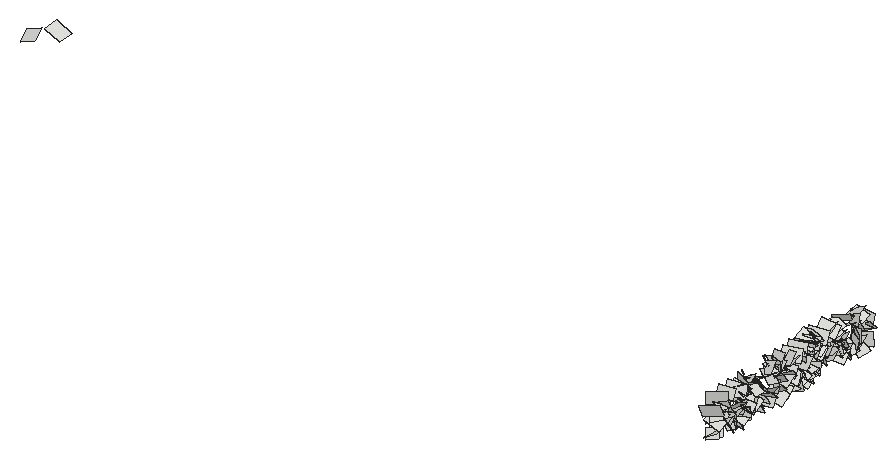
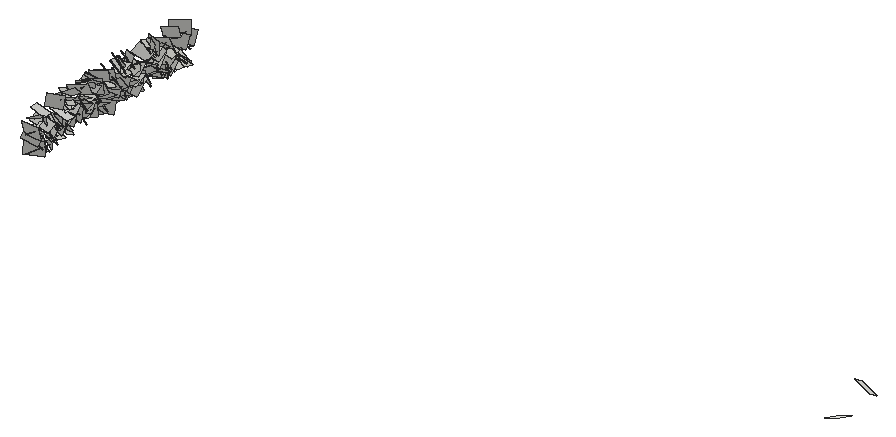
# SketchUp Ruby script. Lengths in inches.
U = 1.inch
M = Sketchup.active_model
def pt(a) = Geom::Point3d.new(a.map { |v| v * U })
def face(e, loops, mat)
  f = e.add_face(loops[0].map { |a| pt(a) })
  loops[1..].each { |l| e.add_face(l.map { |a| pt(a) }).erase! }
  f.material = f.back_material = mat if mat
  f
end
# faces: each face lists its corners as indices into pts; further lists are holes
def faces(e, pts, list, mat = nil) = list.each { |f| face(e, (f[0].is_a?(Array) ? f : [f]).map { |l| l.map { |i| pts[i] } }, mat) }
# xy, xz, yz: faces in a plane at the given z, y or x. An outline is a flat list of corners, or four numbers for a rectangle; further outlines are holes
def ring(l) = l.size == 4 ? [[l[0], l[1]], [l[2], l[1]], [l[2], l[3]], [l[0], l[3]]] : l.each_slice(2).to_a
def flat(e, list, mat, &to3) = list.each { |f| face(e, (f[0].is_a?(Array) ? f : [f]).map { |l| ring(l).map { |u, v| to3.(u, v) } }, mat) }
def xy(e, z, list, mat = nil) = flat(e, list, mat) { |x, y| [x, y, z] }
def xz(e, y, list, mat = nil) = flat(e, list, mat) { |x, z| [x, y, z] }
def yz(e, x, list, mat = nil) = flat(e, list, mat) { |y, z| [x, y, z] }
def lines(e, pts, list) = list.each { |a, b| e.add_line(pt(pts[a]), pt(pts[b])) }
# prism: a flat outline (further loops are holes) pulled along v
def prism(e, loops, v, mat = nil)
  f = face(e, loops, mat); d = Geom::Vector3d.new(v.map { |x| x * U })
  f.pushpull(f.normal.samedirection?(d) ? d.length : -d.length)
end
def box(e, o, s, mat = nil) = prism(e, [[o, [o[0] + s[0], o[1], o[2]], [o[0] + s[0], o[1] + s[1], o[2]], [o[0], o[1] + s[1], o[2]]]], [0, 0, s[2]], mat)
def at(x, y, z, deg = 0) = Geom::Transformation.translation(pt([x, y, z])) * Geom::Transformation.rotation(ORIGIN, Z_AXIS, deg.degrees)
def axes(o, x, y, z) = Geom::Transformation.new([*x, 0, *y, 0, *z, 0, *pt(o).to_a, 1])
def part(name) = M.definitions.add(name)
# library, detail: a bought-in or finely detailed component or shape, given as its bounding box
def library(name, o, s) = part(name).tap { |d| box(d.entities, o, s) }
def detail(e, o, s) = box(e.add_group.entities, o, s)
def put(e, d, t, mat = nil) = e.add_instance(d, t).tap { |i| i.material = mat if mat }
def group(e, t, mat = nil) = e.add_group.tap { |g| g.transformation = t; g.material = mat if mat }.entities
root = M.entities
c1 = part("Component\#6")
p = [[0.01,0,0],[0,3.24,4.54],[4.32,3.24,4.54],[4.33,0,0]]
faces(c1.entities,p,[[0,1,2,3]])
put(root,c1,axes([34.14,183.19,37.72],[0.19709,-1.17807,-0.70591],[0.26547,-0.67132,1.18631],[1.43137,0.28672,-0.12282]))
put(root,c1,axes([34.14,193.54,33.12],[0.22081,1.30446,0.31828],[0.37279,0.25784,-1.28691],[1.3736,-0.27967,0.29809]))
put(root,c1,axes([404.88,193.54,33.12],[-0.22081,1.30446,0.31828],[-0.37279,0.25784,-1.28691],[-1.3736,-0.27967,0.29809]))
put(root,c1,axes([404.88,183.19,37.72],[-0.19709,-1.17807,-0.70591],[-0.26547,-0.67132,1.18631],[-1.43137,0.28672,-0.12282]))
put(root,c1,axes([404.88,179.625,37.91],[-0.28026,0.12179,-1.29213],[-0.26115,-1.29941,-0.07206],[-1.35072,0.22596,0.28204]))
put(root,c1,axes([404.88,128.43,31.91],[-0.33386,1.00192,0.91989],[-0.02581,0.93993,-1.03208],[-1.44154,-0.24887,-0.19457]))
put(root,c1,axes([404.88,132.63,34.3],[-0.186,1.33026,-0.17859],[-0.24164,-0.20703,-1.31812],[-1.40205,-0.1408,0.25087]))
put(root,c1,axes([404.88,206.12,25.83],[-0.28838,0.48251,1.20317],[-0.13396,1.21365,-0.51529],[-1.36755,-0.22063,-0.20324]))
put(root,c1,axes([404.88,163.2,33.68],[-0.16473,-1.2102,0.57798],[-0.2383,0.59712,1.18983],[-1.40149,0.04071,-0.27024]))
put(root,c1,axes([404.88,132.49,21.15],[-0.19066,-0.73145,1.17679],[-0.11238,1.19045,0.72374],[-1.46442,0.00387,-0.20876]))
put(root,c1,axes([404.88,205.05,35.75],[-0.23328,1.34713,-0.22992],[-0.05022,-0.24027,-1.36238],[-1.44774,-0.20874,0.08431]))
put(root,c1,axes([405.22,214.11,35.21],[-0.07772,-0.27644,-1.33377],[-0.91911,-1.02064,0.2592],[-1.11351,0.86175,-0.12086]))
put(root,c1,axes([404.88,141,38.04],[-0.14868,1.2474,-0.57055],[-0.09146,-0.58042,-1.24775],[-1.45112,-0.09122,0.1371]))
put(root,c1,axes([405.59,124.93,30.08],[-0.69154,0.83647,0.57299],[-0.50453,0.34895,-1.05134],[-0.94895,-0.79509,0.14141]))
put(root,c1,axes([404.88,153.14,23.91],[-0.18,-1.08552,0.79109],[-0.08355,0.80406,1.08641],[-1.42134,0.0902,-0.16405]))
put(root,c1,axes([404.88,190.14,35.27],[-0.30668,1.10496,-0.445],[-0.14325,-0.48543,-1.11748],[-1.25452,-0.21469,0.23639]))
put(root,c1,axes([404.88,186.51,25.44],[0.00901,-0.3677,1.34811],[-0.26845,1.32541,0.3631],[-1.45667,-0.24653,-0.05858]))
put(root,c1,axes([404.88,195.625,24.52],[-0.22176,-0.47224,1.18941],[-0.10161,1.2076,0.46259],[-1.3527,-0.0133,-0.22974]))
put(root,c1,axes([404.88,143.09,24.72],[-0.05768,-1.1082,-0.74759],[-0.23067,-0.73089,1.09928],[-1.3981,0.16631,-0.15052]))
put(root,c1,axes([404.88,205.51,24.88],[-0.13882,1.11155,0.63897],[-0.19603,0.6192,-1.11507],[-1.34484,-0.205,0.09658]))
put(root,c1,axes([404.88,157.9,37.93],[-0.24747,1.3445,0.30187],[0.11522,0.32319,-1.35538],[-1.4561,-0.20293,-0.15855]))
put(root,c1,axes([404.88,137.42,26.21],[-0.14568,0.69276,1.17725],[-0.03045,1.18146,-0.69859],[-1.44759,-0.09457,-0.10377]))
put(root,c1,axes([404.88,213.57,27.56],[0.01798,0.03957,-1.39555],[-0.22262,-1.3797,-0.04168],[-1.46303,0.21042,-0.01081]))
put(root,c1,axes([404.88,168.45,29.92],[-0.2904,-0.81126,-1.09363],[0.15157,-1.12651,0.79984],[-1.4354,0.04517,0.30571]))
put(root,c1,axes([404.88,159.18,36.25],[-0.04304,0.74935,1.15311],[-0.14712,1.14549,-0.74928],[-1.45028,-0.13844,0.04179]))
put(root,c1,axes([404.88,165.11,34.6875],[-0.03998,0.77126,1.05992],[-0.2457,1.03973,-0.76482],[-1.36759,-0.20934,0.10642]))
put(root,c1,axes([404.88,200.57,23.13],[-0.2198,-0.69796,1.13548],[0.0671,1.14269,0.71395],[-1.41122,0.16304,-0.1429]))
put(root,c1,axes([404.88,153.125,28.17],[0.03085,-0.9293,0.97672],[-0.26234,0.95667,0.91759],[-1.40479,-0.19906,-0.14991]))
put(root,c1,axes([404.88,172.42,21.79],[-0.22827,-1.35966,0.24048],[0.1567,0.21929,1.3722],[-1.45519,0.2369,0.11004]))
put(root,c1,axes([404.88,122.33,25.2],[-0.14417,1.26196,0.33106],[-0.05821,0.32703,-1.26913],[-1.38172,-0.14545,0.01892]))
put(root,c1,axes([404.88,127.05,26.22],[-0.14417,1.26196,0.33106],[-0.05821,0.32703,-1.26913],[-1.38172,-0.14545,0.01892]))
put(root,c1,axes([404.88,177.28,39.83],[-0.04784,1.11638,-0.64936],[-0.22797,-0.64718,-1.09769],[-1.34988,0.06974,0.20839]))
put(root,c1,axes([404.93,125.55,22.43],[-0.36857,0.54861,0.76203],[-0.54406,0.56941,-0.64413],[-0.83345,-0.61431,0.08349]))
put(root,c1,axes([404.93,123.49,22.43],[-0.36857,0.54861,0.76203],[-0.54406,0.56941,-0.64413],[-0.83345,-0.61431,0.08349]))
put(root,c1,axes([404.88,153.73,28.3],[0.01858,0.99462,-0.84655],[-0.29457,-0.8244,-0.97435],[-1.35277,0.19318,0.20054]))
put(root,c1,axes([404.88,128.45,36.29],[0.02149,0.52903,-1.24729],[-0.2007,-1.23408,-0.5265],[-1.42204,0.18216,0.05546]))
put(root,c1,axes([404.88,124,36.29],[0.02149,0.52903,-1.24729],[-0.2007,-1.23408,-0.5265],[-1.42204,0.18216,0.05546]))
put(root,c1,axes([404.88,128.47,40.0625],[-0.15368,0.21217,-1.35934],[0.08132,-1.3635,-0.221],[-1.45608,-0.09854,0.13113]))
put(root,c1,axes([404.88,188.1875,39.24],[-0.00053,-0.50504,-1.25708],[-0.1621,-1.24903,0.50186],[-1.42684,0.14209,-0.05655]))
put(root,c1,axes([404.88,199.97,41.09],[-0.2759,0.65189,-0.94787],[-0.07756,-0.97924,-0.65337],[-1.21695,-0.08538,0.25653]))
put(root,c1,axes([404.88,183.77,26.5],[-0.0762,-1.33255,-0.21023],[-0.04546,-0.20817,1.33413],[-1.42926,0.07766,-0.03122]))
put(root,c1,axes([404.88,140.4,37.84],[0.00777,-0.46206,-1.23937],[-0.21731,-1.22481,0.45542],[-1.38512,0.18957,-0.0784]))
put(root,c1,axes([404.88,193.84,30.46],[-0.25587,-1.06575,0.3461],[-0.15582,0.3811,1.07099],[-1.17751,0.18115,-0.21693]))
put(root,c1,axes([404.88,194.52,25.48],[-0.11423,-0.20624,1.26777],[-0.06819,1.2715,0.20138],[-1.3598,-0.04643,-0.1166]))
put(root,c1,axes([404.88,189.88,26.35],[-0.12674,1.17916,0.69894],[0.07675,0.70605,-1.17877],[-1.45096,-0.06565,-0.1234]))
put(root,c1,axes([404.88,142.63,35.02],[-0.11092,-0.98462,-0.77371],[-0.1183,-0.76598,0.98988],[-1.32209,0.15114,-0.02366]))
put(root,c1,axes([404.88,142.42,32.89],[-0.18672,-0.42722,1.28431],[0.1337,1.28432,0.44452],[-1.42847,0.17605,-0.12627]))
put(root,c1,axes([404.88,177.96,25.04],[-0.10915,-1.1796,-0.55067],[-0.03689,-0.5497,1.18402],[-1.37942,0.10803,0.01191]))
put(root,c1,axes([404.88,133.32,22.11],[-0.03082,0.0656,1.39488],[0.001,1.39518,-0.0656],[-1.48021,-0.00042,-0.02909]))
put(root,c1,axes([404.88,161.74,34.71],[-0.1652,-1.10091,-0.16395],[-0.26327,-0.12698,1.08875],[-1.15009,0.1872,-0.22568]))
put(root,c1,axes([404.88,211.92,20.51],[-0.20622,-1.25394,-0.15944],[0.06822,-0.17093,1.26581],[-1.33814,0.18453,0.0891]))
put(root,c1,axes([404.88,204.65,33.57],[-0.11682,0.36237,1.1463],[-0.15256,1.13885,-0.37385],[-1.26518,-0.17079,-0.06076]))
put(root,c1,axes([404.88,157.5625,26.25],[-0.15158,-0.38022,-1.22414],[0.0526,-1.23246,0.37701],[-1.35773,-0.0053,0.15127]))
put(root,c1,axes([404.88,135.17,32.61],[-0.12448,1.21649,-0.63228],[0.14654,-0.62086,-1.22019],[-1.44585,-0.16766,-0.06923]))
put(root,c1,axes([404.88,175.66,39.88],[0.03914,-0.32872,-1.22009],[-0.25418,-1.20026,0.31612],[-1.31508,0.2222,-0.09741]))
put(root,c1,axes([404.88,205.46,24.09],[-0.08024,0.04196,1.34674],[0.06239,1.34768,-0.03868],[-1.42687,0.05657,-0.07742]))
put(root,c1,axes([404.88,158.06,26.05],[-0.19995,0.52409,1.06255],[-0.00833,1.07535,-0.5318],[-1.25583,-0.09057,-0.16565]))
put(root,c1,axes([404.88,166.62,31.96],[-0.21061,0.75098,-0.921],[0.02022,-0.93165,-0.76377],[-1.25951,-0.14053,0.14175]))
put(root,c1,axes([404.88,139.39,34.34],[-0.15089,0.92592,0.71699],[-0.08883,0.71236,-0.93659],[-1.23815,-0.16395,-0.02018]))
put(root,c1,axes([404.88,196.54,35.06],[-0.17609,-1.11494,-0.45613],[0.00034,-0.46049,1.12547],[-1.27691,0.15363,0.0632]))
put(root,c1,axes([404.88,156.14,33.68],[-0.06217,-0.55405,1.15944],[-0.03014,1.16092,0.55332],[-1.36179,-0.0004,-0.06518]))
put(root,c1,axes([404.88,205.63,39.17],[-0.17317,1.06099,0.10432],[-0.22006,0.07185,-1.05594],[-1.10844,-0.18002,0.19334]))
put(root,c1,axes([404.88,153.92,36.42],[-0.14295,0.82362,0.79821],[-0.11339,0.79118,-0.83443],[-1.21047,-0.17138,-0.0161]))
put(root,c1,axes([404.88,140.25,33.3],[0.10371,-0.10781,1.29757],[-0.22808,1.282,0.12274],[-1.36119,-0.22303,0.07829]))
put(root,c1,axes([404.88,180.73,30.67],[-0.05707,0.69485,1.12415],[0.04583,1.1254,-0.69356],[-1.4001,0.00851,-0.06852]))
put(root,c1,axes([404.88,145.83,38.68],[0.04371,1.09164,-0.51046],[-0.28885,-0.48908,-1.06793],[-1.24431,0.15188,0.22998]))
put(root,c1,axes([404.88,199.72,26.12],[0.08735,-0.8928,-1.02237],[-0.07635,-1.02569,0.88989],[-1.43674,0.00023,-0.10945]))
put(root,c1,axes([404.88,169.91,24.28],[0.0494,0.58776,1.07494],[-0.25393,1.05932,-0.56884],[-1.27358,-0.18841,0.15511]))
put(root,c1,axes([404.88,178.68,21.25],[-0.14964,-1.02559,0.91665],[0.24358,0.89093,1.03221],[-1.43757,0.25771,0.07948]))
put(root,c1,axes([404.88,196.35,30.1],[-0.25467,1.00338,0.64071],[0.12934,0.67094,-1.00496],[-1.25528,-0.13443,-0.23354]))
put(root,c1,axes([404.88,158.99,33.95],[-0.09747,0.08794,1.12692],[-0.17247,1.11783,-0.1005],[-1.18568,-0.16983,-0.07802]))
put(root,c1,axes([404.88,188.72,38.18],[-0.108,1.17484,0.54266],[0.09899,0.5496,-1.17232],[-1.36819,-0.05298,-0.12766]))
put(root,c1,axes([404.88,187.26,33.24],[-0.066,-0.95024,-0.64083],[-0.19237,-0.6255,0.94515],[-1.19957,0.15259,-0.11631]))
put(root,c1,axes([404.88,141.15,27.9],[-0.10356,0.25866,-1.08582],[-0.18317,-1.08033,-0.24181],[-1.16891,0.14638,0.13409]))
put(root,c1,axes([404.88,173.53,27.66],[-0.08068,-0.97468,-0.75893],[-0.01331,-0.75972,0.97695],[-1.30935,0.06778,0.03684]))
put(root,c1,axes([404.88,181.61,25.33],[0.14764,0.72138,1.18272],[-0.09804,1.19088,-0.71546],[-1.46521,-0.007,0.16705]))
put(root,c1,axes([404.88,198.29,23.22],[-0.04433,-0.32511,1.32538],[0.126,1.3201,0.32757],[-1.44106,0.12543,-0.01213]))
put(root,c1,axes([404.88,200.75,21.625],[-0.14431,-0.01788,1.13958],[-0.06693,1.14604,0.01044],[-1.20625,-0.06145,-0.13692]))
put(root,c1,axes([404.88,130.13,32.75],[-0.05656,-1.14018,0.16245],[-0.17438,0.16851,1.12862],[-1.20828,0.02906,-0.17049]))
put(root,c1,axes([404.88,184.99,36.41],[-0.13687,-0.99381,0.45239],[-0.15227,0.46704,0.985],[-1.14738,0.05657,-0.18469]))
put(root,c1,axes([404.88,190.5,33.59],[-0.11278,1.05886,-0.21225],[-0.21462,-0.22906,-1.04119],[-1.12442,-0.06248,0.22002]))
put(root,c1,axes([404.88,171.44,26.6],[0.03428,0.27698,-1.26013],[-0.06702,-1.25867,-0.27828],[-1.36598,0.0687,-0.01797]))
put(root,c1,axes([404.88,205.99,22.98],[-0.14358,-1.11124,-0.06865],[-0.09474,-0.05808,1.11649],[-1.17635,0.14031,-0.08154]))
put(root,c1,axes([404.88,172.54,38.57],[0.12011,-0.4932,-1.18141],[-0.20578,-1.17893,0.47355],[-1.34134,0.1367,-0.17844]))
put(root,c1,axes([404.88,178.09,32.9],[-0.18757,-0.47698,-1.21124],[0.23196,-1.21588,0.44684],[-1.36024,-0.14157,0.24323]))
put(root,c1,axes([404.88,134.58,22.11],[-0.07114,-1.22092,0.271],[0.02912,0.26988,1.2227],[-1.32535,0.07146,0.01232]))
put(root,c1,axes([404.88,130.54,25.39],[-0.14552,0.87979,0.74939],[-0.0105,0.75374,-0.8867],[-1.22498,-0.11098,-0.08143]))
put(root,c1,axes([404.88,197.21,31.46],[-0.04455,0.58157,-0.95839],[-0.2239,-0.94599,-0.56478],[-1.16701,0.1593,0.14494]))
put(root,c1,axes([404.88,203.71,22.72],[0.0324,0.32539,1.27516],[-0.00551,1.27553,-0.32536],[-1.39498,0.00251,0.0309]))
put(root,c1,axes([404.88,187.29,32.09],[0.03087,-0.89426,-0.74249],[-0.26998,-0.72958,0.86873],[-1.20212,0.14089,-0.21417]))
put(root,c1,axes([404.88,132.97,26.35],[-0.04012,1.17129,0.65858],[0.12839,0.65914,-1.16531],[-1.41857,0.02653,-0.1241]))
put(root,c1,axes([404.88,198.24,37.08],[-0.15669,-0.99926,-0.19378],[-0.22295,-0.1616,0.99377],[-1.05566,0.18244,-0.18112]))
put(root,c1,axes([404.88,160.96,32.62],[-0.12215,0.75895,-0.88724],[-0.014,-0.89234,-0.7616],[-1.23753,-0.06482,0.09619]))
put(root,c1,axes([404.88,164.92,23.28],[-0.02573,-1.02703,-0.88101],[0.12942,-0.87922,1.02158],[-1.42847,-0.06116,0.10843]))
put(root,c1,axes([404.88,138.04,20.07],[0.12016,-0.9858,0.86253],[-0.12902,0.85408,0.99214],[-1.38246,-0.16539,-0.01763]))
put(root,c1,axes([404.88,178.49,34.59],[-0.00763,1.14917,-0.03145],[-0.21412,-0.03223,-1.13128],[-1.19962,-0.00155,0.20212]))
put(root,c1,axes([404.88,133.17,39.1],[-0.0845,-0.28698,-1.03421],[-0.22383,-1.0126,0.29726],[-1.11545,0.22493,0.0187]))
put(root,c1,axes([404.88,141.71,25.57],[0.24627,-1.07768,0.84944],[-0.21085,0.82598,1.10232],[-1.43917,-0.30542,-0.01615]))
put(root,c1,axes([404.88,128.39,27.01],[-0.01413,-1.13969,-0.35832],[-0.11214,-0.35581,1.13564],[-1.2614,0.04439,-0.09695]))
put(root,c1,axes([404.88,182.31,23.94],[0.04872,-1.30982,0.04089],[-0.01644,0.04037,1.31055],[-1.38898,-0.04642,-0.01408]))
put(root,c1,axes([404.88,186.91,28.91],[0.08475,0.77289,1.06783],[-0.0494,1.07079,-0.77154],[-1.39641,0.00903,0.0921]))
put(root,c1,axes([404.88,165.55,34.43],[0.04885,1.13911,0.54464],[-0.08516,0.54654,-1.13629],[-1.33566,0.00681,0.09237]))
put(root,c1,axes([404.88,166.97,25.06],[0.03339,-0.82276,-0.77538],[-0.30966,-0.75526,0.78954],[-1.15769,0.17829,-0.23355]))
put(root,c1,axes([404.88,174.06,31.875],[-0.08593,-0.00736,1.08266],[-0.18405,1.07173,-0.00571],[-1.1328,-0.17357,-0.0812]))
put(root,c1,axes([404.88,193.85,32.27],[-0.12737,1.17977,-0.33684],[0.1012,-0.32843,-1.18439],[-1.29659,-0.14153,-0.05935]))
put(root,c1,axes([404.88,196.04,25.17],[-0.02819,1.07686,0.22249],[-0.25409,0.21152,-1.05244],[-1.13755,-0.07393,0.22957]))
put(root,c1,axes([404.88,177.97,39.67],[0.02985,0.75948,-0.84861],[-0.27983,-0.8214,-0.74388],[-1.17429,0.21504,0.15569]))
put(root,c1,axes([404.88,159.8,34.2],[0.03301,0.77795,0.85676],[-0.24326,0.8442,-0.75821],[-1.20233,-0.14944,0.17692]))
put(root,c1,axes([404.88,180.07,24.39],[0.06666,-0.76105,0.92501],[-0.21989,0.90537,0.75899],[-1.25053,-0.19976,-0.08415]))
put(root,c1,axes([404.88,141.72,37.36],[-0.19445,0.97106,0.50245],[0.00165,0.50971,-0.98451],[-1.15895,-0.1622,-0.0857]))
put(root,c1,axes([404.88,194.3,32.47],[0.23408,0.14056,-1.33491],[-0.22407,-1.33233,-0.17526],[-1.40507,0.23589,-0.19445]))
put(root,c1,axes([404.88,211.85,35.53],[-0.11979,-0.95717,-0.48165],[-0.13908,-0.46832,0.96146],[-1.12727,0.15949,-0.06744]))
put(root,c1,axes([404.88,149.67,23.37],[0.09539,-0.59855,1.14231],[-0.08783,1.14003,0.60389],[-1.36418,-0.11525,0.041]))
put(root,c1,axes([404.88,211.375,32.78],[0.08242,0.8278,-0.94283],[-0.12426,-0.93571,-0.83122],[-1.32412,0.13934,0.01932]))
put(root,c1,axes([404.88,182.77,28.7],[0.0358,-0.11408,-1.31406],[0.04325,-1.31377,0.1151],[-1.39747,-0.04358,-0.0301]))
put(root,c1,axes([404.88,149.48,27.53],[-0.05839,-0.93868,-0.8352],[0.07486,-0.83699,0.93604],[-1.32974,-0.0059,0.08937]))
put(root,c1,axes([404.88,145.76,27.48],[-0.11303,-0.66031,-0.96553],[0.02355,-0.9705,0.66125],[-1.23968,0.04176,0.1006]))
put(root,c1,axes([404.88,169.63,32.59],[-0.01533,-0.4611,-1.03377],[-0.17767,-1.02158,0.45801],[-1.18663,0.15892,-0.05522]))
put(root,c1,axes([404.88,213.71,29.11],[0.07729,-1.24842,0.49404],[0.03127,0.49613,1.24937],[-1.42283,-0.05691,0.0543]))
put(root,c1,axes([404.88,141.59,27.99],[0.06396,0.08339,-1.32201],[0.02487,-1.32324,-0.0824],[-1.4039,-0.01964,-0.06169]))
put(root,c1,axes([404.88,150.86,30.47],[-0.14962,-1.13409,-0.09371],[0.03493,-0.09847,1.14197],[-1.20573,0.13788,0.04471]))
put(root,c1,axes([404.88,179.04,23.77],[-0.11323,-0.75693,-0.7774],[-0.09292,-0.77258,0.76428],[-1.14637,0.13739,0.01483]))
put(root,c1,axes([404.88,188.57,34.3],[0.02784,1.05016,0.5271],[-0.1514,0.52617,-1.0412],[-1.23628,-0.04079,0.13938]))
put(root,c1,axes([404.88,183.25,38.77],[0.07927,-0.40868,-1.12281],[-0.1988,-1.11508,0.39337],[-1.25087,0.15132,-0.13368]))
put(root,c1,axes([404.88,150.2,21.48],[-0.03659,-0.96074,0.6365],[-0.08804,0.6372,0.9573],[-1.21843,-0.01719,-0.08829]))
put(root,c1,axes([404.88,152.25,36.24],[0.0137,1.21221,-0.26433],[-0.01965,-0.26413,-1.21218],[-1.31499,0.01657,0.01536]))
put(root,c1,axes([404.88,158.37,30.5],[-0.12568,-1.12455,0.31778],[0.06348,0.31314,1.13049],[-1.23707,0.13032,0.02572]))
put(root,c1,axes([404.88,160.22,28.4],[-0.15479,0.80897,-0.76348],[0.02106,-0.76802,-0.81757],[-1.17891,-0.11994,0.08565]))
put(root,c1,axes([404.88,144,25.2],[-0.04504,0.58566,0.95802],[-0.11757,0.95183,-0.5868],[-1.18441,-0.11675,0.02182]))
put(root,c1,axes([404.88,143.97,23.32],[-0.18437,0.48358,0.83906],[-0.16998,0.82633,-0.50949],[-1.01237,-0.22682,-0.06726]))
put(root,c1,axes([404.88,197.73,24.08],[-0.06299,0.80841,0.87356],[0.01823,0.87514,-0.8087],[-1.26151,-0.02772,-0.0553]))
put(root,c1,axes([404.88,194.96,38.36],[0.08597,-0.96025,-0.92678],[0.03419,-0.92681,0.9631],[-1.41421,-0.08078,-0.03305]))
put(root,c1,axes([404.88,142.6875,32.73],[0.11413,-1.14483,0.29443],[-0.2702,0.26621,1.12831],[-1.22353,-0.16558,-0.2217]))
